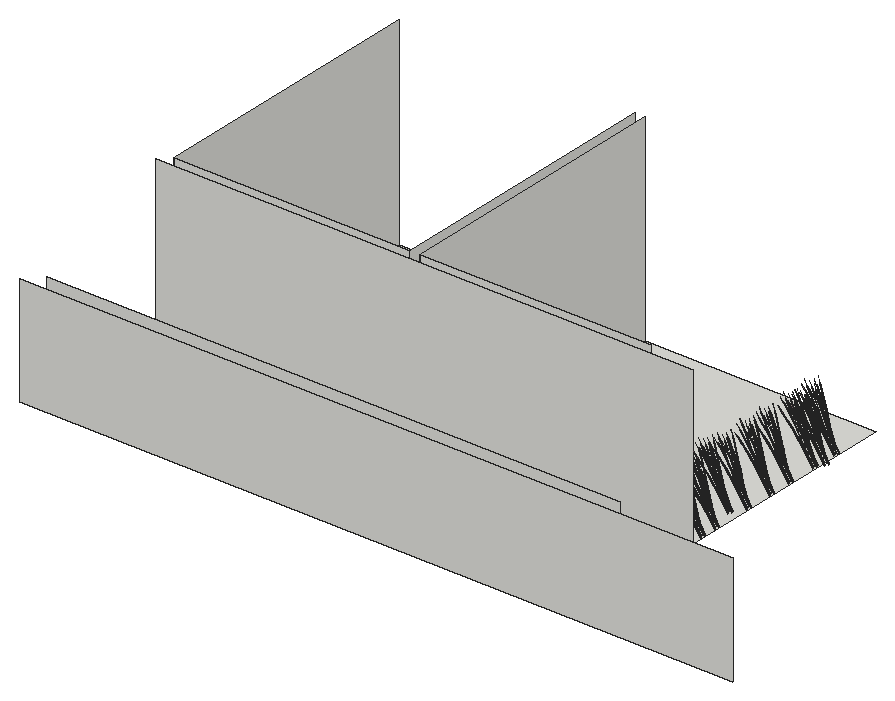
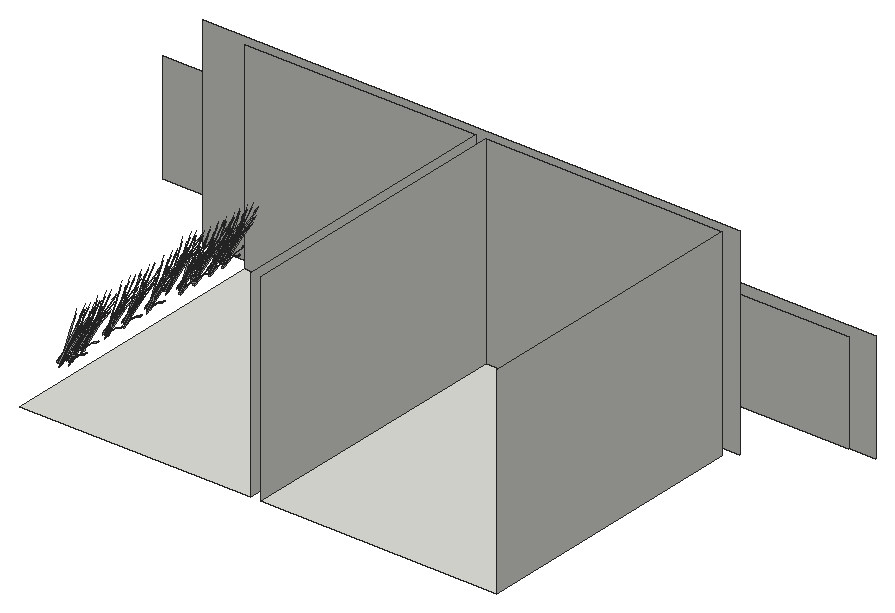
# SketchUp Ruby script. Lengths in inches.
U = 1.inch
M = Sketchup.active_model
def pt(a) = Geom::Point3d.new(a.map { |v| v * U })
def face(e, loops, mat)
  f = e.add_face(loops[0].map { |a| pt(a) })
  loops[1..].each { |l| e.add_face(l.map { |a| pt(a) }).erase! }
  f.material = f.back_material = mat if mat
  f
end
# faces: each face lists its corners as indices into pts; further lists are holes
def faces(e, pts, list, mat = nil) = list.each { |f| face(e, (f[0].is_a?(Array) ? f : [f]).map { |l| l.map { |i| pts[i] } }, mat) }
# xy, xz, yz: faces in a plane at the given z, y or x. An outline is a flat list of corners, or four numbers for a rectangle; further outlines are holes
def ring(l) = l.size == 4 ? [[l[0], l[1]], [l[2], l[1]], [l[2], l[3]], [l[0], l[3]]] : l.each_slice(2).to_a
def flat(e, list, mat, &to3) = list.each { |f| face(e, (f[0].is_a?(Array) ? f : [f]).map { |l| ring(l).map { |u, v| to3.(u, v) } }, mat) }
def xy(e, z, list, mat = nil) = flat(e, list, mat) { |x, y| [x, y, z] }
def xz(e, y, list, mat = nil) = flat(e, list, mat) { |x, z| [x, y, z] }
def yz(e, x, list, mat = nil) = flat(e, list, mat) { |y, z| [x, y, z] }
def lines(e, pts, list) = list.each { |a, b| e.add_line(pt(pts[a]), pt(pts[b])) }
# prism: a flat outline (further loops are holes) pulled along v
def prism(e, loops, v, mat = nil)
  f = face(e, loops, mat); d = Geom::Vector3d.new(v.map { |x| x * U })
  f.pushpull(f.normal.samedirection?(d) ? d.length : -d.length)
end
def box(e, o, s, mat = nil) = prism(e, [[o, [o[0] + s[0], o[1], o[2]], [o[0] + s[0], o[1] + s[1], o[2]], [o[0], o[1] + s[1], o[2]]]], [0, 0, s[2]], mat)
def at(x, y, z, deg = 0) = Geom::Transformation.translation(pt([x, y, z])) * Geom::Transformation.rotation(ORIGIN, Z_AXIS, deg.degrees)
def axes(o, x, y, z) = Geom::Transformation.new([*x, 0, *y, 0, *z, 0, *pt(o).to_a, 1])
def part(name) = M.definitions.add(name)
# library, detail: a bought-in or finely detailed component or shape, given as its bounding box
def library(name, o, s) = part(name).tap { |d| box(d.entities, o, s) }
def detail(e, o, s) = box(e.add_group.entities, o, s)
def put(e, d, t, mat = nil) = e.add_instance(d, t).tap { |i| i.material = mat if mat }
def group(e, t, mat = nil) = e.add_group.tap { |g| g.transformation = t; g.material = mat if mat }.entities
root = M.entities
M.materials.add("LightPink_Translucent").color = [144, 107, 117]
M.materials["LightPink_Translucent"].alpha = 0.75
c1 = part("blade")
p = [[2.15,0.21,22],[0,0.17,0],[0.09,0.45,0],[2.18,0.31,22],[2.29,0.31,22],[0.38,0.45,0],
  [2.48,0.24,33],[2.49,0.24,33],[2.48,0.22,33]]
faces(c1.entities,p,[[0,1,2,3],[4,5,2,3],[6,3,4,7],[8,0,3,6]])
c2 = part("seeds")
p = [[0.3,-0.1,1.38],[-0.01,-0.03,1.59],[-0.01,-0.03,0.03],[0.14,-0.07,-0.07],[0.29,-0.03,3],[0.15,0.01,3.11]]
faces(c2.entities,p,[[0,1,2,3],[1,0,4,5]],"LightPink_Translucent")
c3 = part("blade with seeds")
put(c3.entities,c1,at(0,0,0))
put(c3.entities,c2,axes([2.4,0.25,30.99],[1.5799,-0.05474,1.17369],[-0.12525,1.92788,0.29478],[-0.07173,-0.02425,1.56792]))
xy(root,0,[[51,51,192,219],[198,51,336,219]])
xz(root,0,[[0,-6,426,60]])
xz(root,9,[[9,0,351,60]])
xz(root,45,[[45,0,366,120]])
xz(root,51,[[51,0,192,120],[198,0,336,120]])
yz(root,51,[[51,0,219,120]])
yz(root,192,[[51,0,219,120]])
yz(root,198,[[51,0,219,120]])
put(root,c3,axes([340.35,60.81,6.17],[0.37107,-0.01478,1.71376],[-0.24616,0.64047,0.13857],[-0.5288,-0.03961,0.73262]))
put(root,c3,axes([340.35,70.63,6.17],[0.37107,-0.01478,1.71376],[-0.24616,0.64047,0.13857],[-0.5288,-0.03961,0.73262]))
put(root,c3,axes([340.35,82.63,6.17],[0.37107,-0.01478,1.71376],[-0.24616,0.64047,0.13857],[-0.5288,-0.03961,0.73262]))
put(root,c3,axes([340.35,93.1,6.17],[0.37107,-0.01478,1.71376],[-0.24616,0.64047,0.13857],[-0.5288,-0.03961,0.73262]))
put(root,c3,axes([340.35,103.17,9.875],[0.37107,-0.01478,1.71376],[-0.24616,0.64047,0.13857],[-0.5288,-0.03961,0.73262]))
put(root,c3,axes([340.35,117.18,6.17],[0.37107,-0.01478,1.71376],[-0.24616,0.64047,0.13857],[-0.5288,-0.03961,0.73262]))
put(root,c3,axes([340.35,134.12,6.17],[0.37107,-0.01478,1.71376],[-0.24616,0.64047,0.13857],[-0.5288,-0.03961,0.73262]))
put(root,c3,axes([340.35,148.47,6.17],[0.37107,-0.01478,1.71376],[-0.24616,0.64047,0.13857],[-0.5288,-0.03961,0.73262]))
put(root,c3,axes([340.35,166.63,6.17],[0.37107,-0.01478,1.71376],[-0.24616,0.64047,0.13857],[-0.5288,-0.03961,0.73262]))
put(root,c3,axes([340.35,175.28,3.875],[0.37107,-0.01478,1.71376],[-0.24616,0.64047,0.13857],[-0.5288,-0.03961,0.73262]))
put(root,c3,axes([340.35,182.45,6.17],[0.37107,-0.01478,1.71376],[-0.24616,0.64047,0.13857],[-0.5288,-0.03961,0.73262]))
put(root,c3,axes([340.51,61.93,6.17],[0.31041,-0.13801,1.71376],[0.26133,0.63772,0.13857],[-0.48731,0.14413,0.73262]))
put(root,c3,axes([340.51,71.76,6.17],[0.31041,-0.13801,1.71376],[0.26133,0.63772,0.13857],[-0.48731,0.14413,0.73262]))
put(root,c3,axes([340.51,83.76,6.17],[0.31041,-0.13801,1.71376],[0.26133,0.63772,0.13857],[-0.48731,0.14413,0.73262]))
put(root,c3,axes([340.51,94.23,6.17],[0.31041,-0.13801,1.71376],[0.26133,0.63772,0.13857],[-0.48731,0.14413,0.73262]))
put(root,c3,axes([340.51,104.3,9.875],[0.31041,-0.13801,1.71376],[0.26133,0.63772,0.13857],[-0.48731,0.14413,0.73262]))
put(root,c3,axes([340.51,118.31,6.17],[0.31041,-0.13801,1.71376],[0.26133,0.63772,0.13857],[-0.48731,0.14413,0.73262]))
put(root,c3,axes([340.51,135.25,6.17],[0.31041,-0.13801,1.71376],[0.26133,0.63772,0.13857],[-0.48731,0.14413,0.73262]))
put(root,c3,axes([340.51,149.59,6.17],[0.31041,-0.13801,1.71376],[0.26133,0.63772,0.13857],[-0.48731,0.14413,0.73262]))
put(root,c3,axes([340.51,167.76,6.17],[0.31041,-0.13801,1.71376],[0.26133,0.63772,0.13857],[-0.48731,0.14413,0.73262]))
put(root,c3,axes([340.51,176.41,3.875],[0.31041,-0.13801,1.71376],[0.26133,0.63772,0.13857],[-0.48731,0.14413,0.73262]))
put(root,c3,axes([340.51,183.58,6.17],[0.31041,-0.13801,1.71376],[0.26133,0.63772,0.13857],[-0.48731,0.14413,0.73262]))
put(root,c3,axes([339.54,63.02,4.88],[0.3109,0.05356,1.43002],[0.20038,0.54709,-0.30754],[-0.42231,0.10241,0.61141]))
put(root,c3,axes([339.54,72.85,4.88],[0.3109,0.05356,1.43002],[0.20038,0.54709,-0.30754],[-0.42231,0.10241,0.61141]))
put(root,c3,axes([339.54,84.85,4.88],[0.3109,0.05356,1.43002],[0.20038,0.54709,-0.30754],[-0.42231,0.10241,0.61141]))
put(root,c3,axes([339.54,95.32,4.88],[0.3109,0.05356,1.43002],[0.20038,0.54709,-0.30754],[-0.42231,0.10241,0.61141]))
put(root,c3,axes([339.54,105.39,8.59],[0.3109,0.05356,1.43002],[0.20038,0.54709,-0.30754],[-0.42231,0.10241,0.61141]))
put(root,c3,axes([339.54,119.39,4.88],[0.3109,0.05356,1.43002],[0.20038,0.54709,-0.30754],[-0.42231,0.10241,0.61141]))
put(root,c3,axes([339.54,136.33,4.88],[0.3109,0.05356,1.43002],[0.20038,0.54709,-0.30754],[-0.42231,0.10241,0.61141]))
put(root,c3,axes([339.54,150.68,4.88],[0.3109,0.05356,1.43002],[0.20038,0.54709,-0.30754],[-0.42231,0.10241,0.61141]))
put(root,c3,axes([339.54,168.85,4.88],[0.3109,0.05356,1.43002],[0.20038,0.54709,-0.30754],[-0.42231,0.10241,0.61141]))
put(root,c3,axes([339.54,177.5,2.59],[0.3109,0.05356,1.43002],[0.20038,0.54709,-0.30754],[-0.42231,0.10241,0.61141]))
put(root,c3,axes([339.54,184.67,4.88],[0.3109,0.05356,1.43002],[0.20038,0.54709,-0.30754],[-0.42231,0.10241,0.61141]))
put(root,c3,axes([342.29,61.27,5.63],[0.25429,-0.09438,1.77064],[0.08769,0.65901,0.13857],[-0.5508,0.08745,0.63284]))
put(root,c3,axes([342.29,71.09,5.63],[0.25429,-0.09438,1.77064],[0.08769,0.65901,0.13857],[-0.5508,0.08745,0.63284]))
put(root,c3,axes([342.29,83.09,5.63],[0.25429,-0.09438,1.77064],[0.08769,0.65901,0.13857],[-0.5508,0.08745,0.63284]))
put(root,c3,axes([342.29,93.57,5.63],[0.25429,-0.09438,1.77064],[0.08769,0.65901,0.13857],[-0.5508,0.08745,0.63284]))
put(root,c3,axes([342.29,103.63,9.34],[0.25429,-0.09438,1.77064],[0.08769,0.65901,0.13857],[-0.5508,0.08745,0.63284]))
put(root,c3,axes([342.29,117.64,5.63],[0.25429,-0.09438,1.77064],[0.08769,0.65901,0.13857],[-0.5508,0.08745,0.63284]))
put(root,c3,axes([342.29,134.58,5.63],[0.25429,-0.09438,1.77064],[0.08769,0.65901,0.13857],[-0.5508,0.08745,0.63284]))
put(root,c3,axes([342.29,148.93,5.63],[0.25429,-0.09438,1.77064],[0.08769,0.65901,0.13857],[-0.5508,0.08745,0.63284]))
put(root,c3,axes([342.29,167.09,5.63],[0.25429,-0.09438,1.77064],[0.08769,0.65901,0.13857],[-0.5508,0.08745,0.63284]))
put(root,c3,axes([342.29,175.75,3.34],[0.25429,-0.09438,1.77064],[0.08769,0.65901,0.13857],[-0.5508,0.08745,0.63284]))
put(root,c3,axes([342.29,182.91,5.63],[0.25429,-0.09438,1.77064],[0.08769,0.65901,0.13857],[-0.5508,0.08745,0.63284]))
put(root,c3,axes([339.56,61.71,7.01],[-0.14609,0.08471,1.74944],[0.01243,0.61893,-0.27667],[-0.33486,0.08049,0.14031]))
put(root,c3,axes([339.56,71.54,7.01],[-0.14609,0.08471,1.74944],[0.01243,0.61893,-0.27667],[-0.33486,0.08049,0.14031]))
put(root,c3,axes([339.56,83.54,7.01],[-0.14609,0.08471,1.74944],[0.01243,0.61893,-0.27667],[-0.33486,0.08049,0.14031]))
put(root,c3,axes([339.56,94.01,7.01],[-0.14609,0.08471,1.74944],[0.01243,0.61893,-0.27667],[-0.33486,0.08049,0.14031]))
put(root,c3,axes([339.56,118.08,7.01],[-0.14609,0.08471,1.74944],[0.01243,0.61893,-0.27667],[-0.33486,0.08049,0.14031]))
put(root,c3,axes([339.56,135.02,7.01],[-0.14609,0.08471,1.74944],[0.01243,0.61893,-0.27667],[-0.33486,0.08049,0.14031]))
put(root,c3,axes([339.56,149.37,7.01],[-0.14609,0.08471,1.74944],[0.01243,0.61893,-0.27667],[-0.33486,0.08049,0.14031]))
put(root,c3,axes([339.56,167.53,7.01],[-0.14609,0.08471,1.74944],[0.01243,0.61893,-0.27667],[-0.33486,0.08049,0.14031]))
put(root,c3,axes([339.56,176.1875,4.72],[-0.14609,0.08471,1.74944],[0.01243,0.61893,-0.27667],[-0.33486,0.08049,0.14031]))
put(root,c3,axes([339.56,183.36,7.01],[-0.14609,0.08471,1.74944],[0.01243,0.61893,-0.27667],[-0.33486,0.08049,0.14031]))
put(root,c3,axes([341.46,60.21,7.27],[-0.89428,-0.01571,-0.71045],[0.06006,-0.66153,0.08574],[-0.37886,-0.06981,1.00501]))
put(root,c3,axes([341.46,70.04,7.27],[-0.89428,-0.01571,-0.71045],[0.06006,-0.66153,0.08574],[-0.37886,-0.06981,1.00501]))
put(root,c3,axes([341.46,82.04,7.27],[-0.89428,-0.01571,-0.71045],[0.06006,-0.66153,0.08574],[-0.37886,-0.06981,1.00501]))
put(root,c3,axes([341.46,92.51,7.27],[-0.89428,-0.01571,-0.71045],[0.06006,-0.66153,0.08574],[-0.37886,-0.06981,1.00501]))
put(root,c3,axes([341.46,102.58,10.98],[-0.89428,-0.01571,-0.71045],[0.06006,-0.66153,0.08574],[-0.37886,-0.06981,1.00501]))
put(root,c3,axes([341.46,116.58,7.27],[-0.89428,-0.01571,-0.71045],[0.06006,-0.66153,0.08574],[-0.37886,-0.06981,1.00501]))
put(root,c3,axes([341.46,133.52,7.27],[-0.89428,-0.01571,-0.71045],[0.06006,-0.66153,0.08574],[-0.37886,-0.06981,1.00501]))
put(root,c3,axes([341.46,147.87,7.27],[-0.89428,-0.01571,-0.71045],[0.06006,-0.66153,0.08574],[-0.37886,-0.06981,1.00501]))
put(root,c3,axes([341.46,166.04,7.27],[-0.89428,-0.01571,-0.71045],[0.06006,-0.66153,0.08574],[-0.37886,-0.06981,1.00501]))
put(root,c3,axes([341.46,174.69,4.98],[-0.89428,-0.01571,-0.71045],[0.06006,-0.66153,0.08574],[-0.37886,-0.06981,1.00501]))
put(root,c3,axes([341.46,181.86,7.27],[-0.89428,-0.01571,-0.71045],[0.06006,-0.66153,0.08574],[-0.37886,-0.06981,1.00501]))
put(root,c3,axes([340.74,60.37,4.88],[0.17466,0.18165,1.43002],[-0.40248,0.49377,-0.30754],[-0.41327,-0.11802,0.61141]))
put(root,c3,axes([340.74,70.2,4.88],[0.17466,0.18165,1.43002],[-0.40248,0.49377,-0.30754],[-0.41327,-0.11802,0.61141]))
put(root,c3,axes([340.74,82.2,4.88],[0.17466,0.18165,1.43002],[-0.40248,0.49377,-0.30754],[-0.41327,-0.11802,0.61141]))
put(root,c3,axes([340.74,92.67,4.88],[0.17466,0.18165,1.43002],[-0.40248,0.49377,-0.30754],[-0.41327,-0.11802,0.61141]))
put(root,c3,axes([340.74,102.74,8.59],[0.17466,0.18165,1.43002],[-0.40248,0.49377,-0.30754],[-0.41327,-0.11802,0.61141]))
put(root,c3,axes([340.74,116.75,4.88],[0.17466,0.18165,1.43002],[-0.40248,0.49377,-0.30754],[-0.41327,-0.11802,0.61141]))
put(root,c3,axes([340.74,133.6875,4.88],[0.17466,0.18165,1.43002],[-0.40248,0.49377,-0.30754],[-0.41327,-0.11802,0.61141]))
put(root,c3,axes([340.74,148.03,4.88],[0.17466,0.18165,1.43002],[-0.40248,0.49377,-0.30754],[-0.41327,-0.11802,0.61141]))
put(root,c3,axes([340.74,166.2,4.88],[0.17466,0.18165,1.43002],[-0.40248,0.49377,-0.30754],[-0.41327,-0.11802,0.61141]))
put(root,c3,axes([340.74,174.85,2.59],[0.17466,0.18165,1.43002],[-0.40248,0.49377,-0.30754],[-0.41327,-0.11802,0.61141]))
put(root,c3,axes([340.74,182.02,4.88],[0.17466,0.18165,1.43002],[-0.40248,0.49377,-0.30754],[-0.41327,-0.11802,0.61141]))
put(root,c3,axes([340.03,61.36,6.82],[-0.74348,-0.18202,-0.35414],[0.21685,-0.53102,0.4572],[-0.29933,0.04869,0.87481]))
put(root,c3,axes([340.03,71.18,6.82],[-0.74348,-0.18202,-0.35414],[0.21685,-0.53102,0.4572],[-0.29933,0.04869,0.87481]))
put(root,c3,axes([340.03,83.18,6.82],[-0.74348,-0.18202,-0.35414],[0.21685,-0.53102,0.4572],[-0.29933,0.04869,0.87481]))
put(root,c3,axes([340.03,93.65,6.82],[-0.74348,-0.18202,-0.35414],[0.21685,-0.53102,0.4572],[-0.29933,0.04869,0.87481]))
put(root,c3,axes([340.03,103.72,10.53],[-0.74348,-0.18202,-0.35414],[0.21685,-0.53102,0.4572],[-0.29933,0.04869,0.87481]))
put(root,c3,axes([340.03,117.73,6.82],[-0.74348,-0.18202,-0.35414],[0.21685,-0.53102,0.4572],[-0.29933,0.04869,0.87481]))
put(root,c3,axes([340.03,134.67,6.82],[-0.74348,-0.18202,-0.35414],[0.21685,-0.53102,0.4572],[-0.29933,0.04869,0.87481]))
put(root,c3,axes([340.03,149.02,6.82],[-0.74348,-0.18202,-0.35414],[0.21685,-0.53102,0.4572],[-0.29933,0.04869,0.87481]))
put(root,c3,axes([340.03,167.18,6.82],[-0.74348,-0.18202,-0.35414],[0.21685,-0.53102,0.4572],[-0.29933,0.04869,0.87481]))
put(root,c3,axes([340.03,175.84,4.53],[-0.74348,-0.18202,-0.35414],[0.21685,-0.53102,0.4572],[-0.29933,0.04869,0.87481]))
put(root,c3,axes([340.03,183,6.82],[-0.74348,-0.18202,-0.35414],[0.21685,-0.53102,0.4572],[-0.29933,0.04869,0.87481]))
put(root,c3,axes([341.05,59.78,6.17],[0.3323,0.11241,1.71376],[-0.68769,0.4716,0.13857],[-0.42861,-0.21275,0.73262]))
put(root,c3,axes([341.05,69.61,6.17],[0.3323,0.11241,1.71376],[-0.68769,0.4716,0.13857],[-0.42861,-0.21275,0.73262]))
put(root,c3,axes([341.05,81.61,6.17],[0.3323,0.11241,1.71376],[-0.68769,0.4716,0.13857],[-0.42861,-0.21275,0.73262]))
put(root,c3,axes([341.05,92.08,6.17],[0.3323,0.11241,1.71376],[-0.68769,0.4716,0.13857],[-0.42861,-0.21275,0.73262]))
put(root,c3,axes([341.05,102.14,9.875],[0.3323,0.11241,1.71376],[-0.68769,0.4716,0.13857],[-0.42861,-0.21275,0.73262]))
put(root,c3,axes([341.05,116.15,6.17],[0.3323,0.11241,1.71376],[-0.68769,0.4716,0.13857],[-0.42861,-0.21275,0.73262]))
put(root,c3,axes([341.05,133.09,6.17],[0.3323,0.11241,1.71376],[-0.68769,0.4716,0.13857],[-0.42861,-0.21275,0.73262]))
put(root,c3,axes([341.05,147.4375,6.17],[0.3323,0.11241,1.71376],[-0.68769,0.4716,0.13857],[-0.42861,-0.21275,0.73262]))
put(root,c3,axes([341.05,165.6,6.17],[0.3323,0.11241,1.71376],[-0.68769,0.4716,0.13857],[-0.42861,-0.21275,0.73262]))
put(root,c3,axes([341.05,174.26,3.875],[0.3323,0.11241,1.71376],[-0.68769,0.4716,0.13857],[-0.42861,-0.21275,0.73262]))
put(root,c3,axes([341.05,181.43,6.17],[0.3323,0.11241,1.71376],[-0.68769,0.4716,0.13857],[-0.42861,-0.21275,0.73262]))
put(root,c3,axes([337.93,62.34,7],[0.11417,0.0175,1.77383],[0.35319,0.57649,-0.16761],[-0.23371,0.15131,0.31391]))
put(root,c3,axes([337.93,72.16,7],[0.11417,0.0175,1.77383],[0.35319,0.57649,-0.16761],[-0.23371,0.15131,0.31391]))
put(root,c3,axes([337.93,84.16,7],[0.11417,0.0175,1.77383],[0.35319,0.57649,-0.16761],[-0.23371,0.15131,0.31391]))
put(root,c3,axes([337.93,94.63,7],[0.11417,0.0175,1.77383],[0.35319,0.57649,-0.16761],[-0.23371,0.15131,0.31391]))
put(root,c3,axes([337.93,118.71,7],[0.11417,0.0175,1.77383],[0.35319,0.57649,-0.16761],[-0.23371,0.15131,0.31391]))
put(root,c3,axes([337.93,135.65,7],[0.11417,0.0175,1.77383],[0.35319,0.57649,-0.16761],[-0.23371,0.15131,0.31391]))
put(root,c3,axes([337.93,150,7],[0.11417,0.0175,1.77383],[0.35319,0.57649,-0.16761],[-0.23371,0.15131,0.31391]))
put(root,c3,axes([337.93,168.16,7],[0.11417,0.0175,1.77383],[0.35319,0.57649,-0.16761],[-0.23371,0.15131,0.31391]))
put(root,c3,axes([337.93,176.8125,4.71],[0.11417,0.0175,1.77383],[0.35319,0.57649,-0.16761],[-0.23371,0.15131,0.31391]))
put(root,c3,axes([337.93,183.98,7],[0.11417,0.0175,1.77383],[0.35319,0.57649,-0.16761],[-0.23371,0.15131,0.31391]))
put(root,c3,axes([340.54,61.63,6.97],[-0.24236,0.59349,-0.51099],[-0.83094,-0.20343,-0.3958],[-0.33455,0.05442,0.97773]))
put(root,c3,axes([340.54,71.45,6.97],[-0.24236,0.59349,-0.51099],[-0.83094,-0.20343,-0.3958],[-0.33455,0.05442,0.97773]))
put(root,c3,axes([340.54,83.45,6.97],[-0.24236,0.59349,-0.51099],[-0.83094,-0.20343,-0.3958],[-0.33455,0.05442,0.97773]))
put(root,c3,axes([340.54,93.92,6.97],[-0.24236,0.59349,-0.51099],[-0.83094,-0.20343,-0.3958],[-0.33455,0.05442,0.97773]))
put(root,c3,axes([340.54,103.99,10.68],[-0.24236,0.59349,-0.51099],[-0.83094,-0.20343,-0.3958],[-0.33455,0.05442,0.97773]))
put(root,c3,axes([340.54,118,6.97],[-0.24236,0.59349,-0.51099],[-0.83094,-0.20343,-0.3958],[-0.33455,0.05442,0.97773]))
put(root,c3,axes([340.54,134.94,6.97],[-0.24236,0.59349,-0.51099],[-0.83094,-0.20343,-0.3958],[-0.33455,0.05442,0.97773]))
put(root,c3,axes([340.54,149.29,6.97],[-0.24236,0.59349,-0.51099],[-0.83094,-0.20343,-0.3958],[-0.33455,0.05442,0.97773]))
put(root,c3,axes([340.54,167.45,6.97],[-0.24236,0.59349,-0.51099],[-0.83094,-0.20343,-0.3958],[-0.33455,0.05442,0.97773]))
put(root,c3,axes([340.54,176.11,4.68],[-0.24236,0.59349,-0.51099],[-0.83094,-0.20343,-0.3958],[-0.33455,0.05442,0.97773]))
put(root,c3,axes([340.54,183.27,6.97],[-0.24236,0.59349,-0.51099],[-0.83094,-0.20343,-0.3958],[-0.33455,0.05442,0.97773]))
put(root,c3,axes([341.17,60.35,6.97],[-0.6496,0.4322,-0.51099],[-0.5689,-0.45657,-0.3958],[-0.33005,-0.06576,0.97773]))
put(root,c3,axes([341.17,70.17,6.97],[-0.6496,0.4322,-0.51099],[-0.5689,-0.45657,-0.3958],[-0.33005,-0.06576,0.97773]))
put(root,c3,axes([341.17,82.17,6.97],[-0.6496,0.4322,-0.51099],[-0.5689,-0.45657,-0.3958],[-0.33005,-0.06576,0.97773]))
put(root,c3,axes([341.17,92.64,6.97],[-0.6496,0.4322,-0.51099],[-0.5689,-0.45657,-0.3958],[-0.33005,-0.06576,0.97773]))
put(root,c3,axes([341.17,102.71,10.68],[-0.6496,0.4322,-0.51099],[-0.5689,-0.45657,-0.3958],[-0.33005,-0.06576,0.97773]))
put(root,c3,axes([341.17,116.72,6.97],[-0.6496,0.4322,-0.51099],[-0.5689,-0.45657,-0.3958],[-0.33005,-0.06576,0.97773]))
put(root,c3,axes([341.17,133.66,6.97],[-0.6496,0.4322,-0.51099],[-0.5689,-0.45657,-0.3958],[-0.33005,-0.06576,0.97773]))
put(root,c3,axes([341.17,148.01,6.97],[-0.6496,0.4322,-0.51099],[-0.5689,-0.45657,-0.3958],[-0.33005,-0.06576,0.97773]))
put(root,c3,axes([341.17,166.17,6.97],[-0.6496,0.4322,-0.51099],[-0.5689,-0.45657,-0.3958],[-0.33005,-0.06576,0.97773]))
put(root,c3,axes([341.17,174.82,4.68],[-0.6496,0.4322,-0.51099],[-0.5689,-0.45657,-0.3958],[-0.33005,-0.06576,0.97773]))
put(root,c3,axes([341.17,181.99,6.97],[-0.6496,0.4322,-0.51099],[-0.5689,-0.45657,-0.3958],[-0.33005,-0.06576,0.97773]))
put(root,c3,axes([340.12,61.59,3.79],[0.02269,0.10283,1.76342],[-0.45738,0.53699,-0.26939],[-0.32488,-0.02707,0.30037]))
put(root,c3,axes([340.12,71.42,3.79],[0.02269,0.10283,1.76342],[-0.45738,0.53699,-0.26939],[-0.32488,-0.02707,0.30037]))
put(root,c3,axes([340.12,83.42,3.79],[0.02269,0.10283,1.76342],[-0.45738,0.53699,-0.26939],[-0.32488,-0.02707,0.30037]))
put(root,c3,axes([340.12,93.89,3.79],[0.02269,0.10283,1.76342],[-0.45738,0.53699,-0.26939],[-0.32488,-0.02707,0.30037]))
